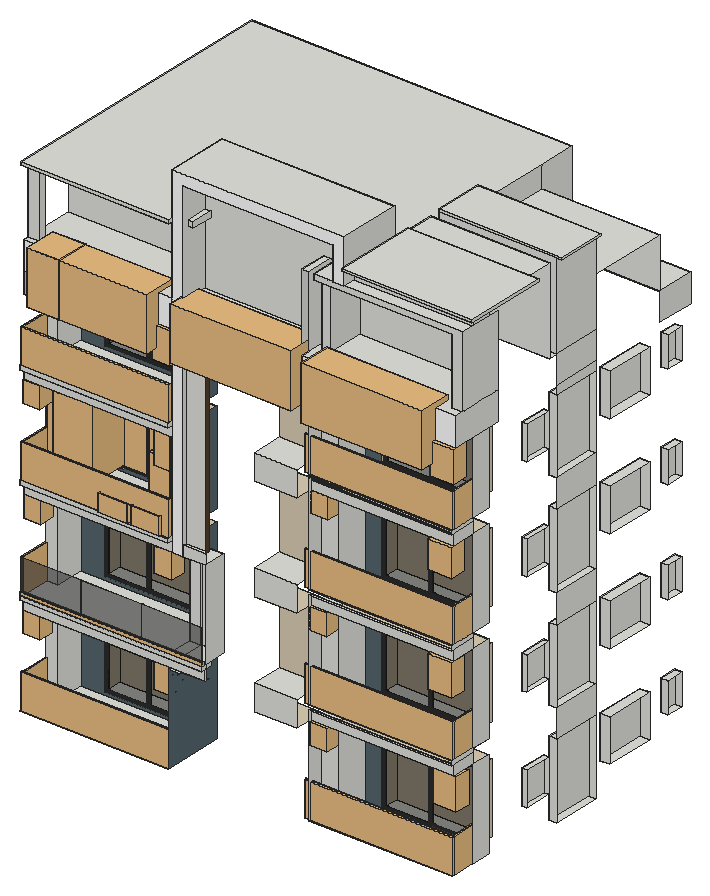
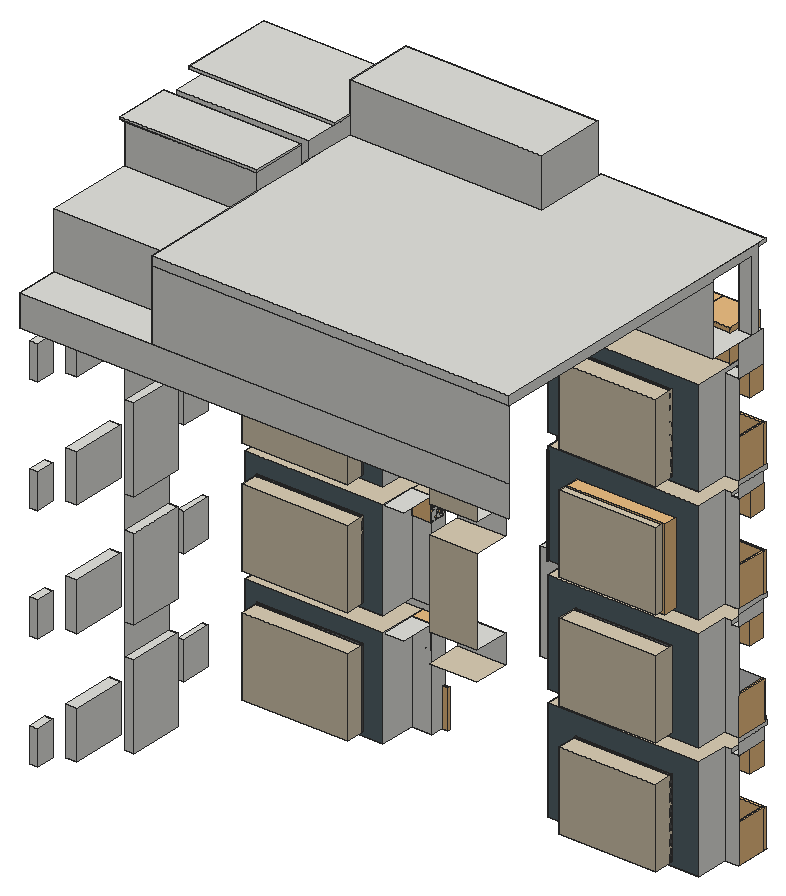
# SketchUp Ruby script. Lengths in inches.
U = 1.inch
M = Sketchup.active_model
def pt(a) = Geom::Point3d.new(a.map { |v| v * U })
def face(e, loops, mat)
  f = e.add_face(loops[0].map { |a| pt(a) })
  loops[1..].each { |l| e.add_face(l.map { |a| pt(a) }).erase! }
  f.material = f.back_material = mat if mat
  f
end
# faces: each face lists its corners as indices into pts; further lists are holes
def faces(e, pts, list, mat = nil) = list.each { |f| face(e, (f[0].is_a?(Array) ? f : [f]).map { |l| l.map { |i| pts[i] } }, mat) }
# xy, xz, yz: faces in a plane at the given z, y or x. An outline is a flat list of corners, or four numbers for a rectangle; further outlines are holes
def ring(l) = l.size == 4 ? [[l[0], l[1]], [l[2], l[1]], [l[2], l[3]], [l[0], l[3]]] : l.each_slice(2).to_a
def flat(e, list, mat, &to3) = list.each { |f| face(e, (f[0].is_a?(Array) ? f : [f]).map { |l| ring(l).map { |u, v| to3.(u, v) } }, mat) }
def xy(e, z, list, mat = nil) = flat(e, list, mat) { |x, y| [x, y, z] }
def xz(e, y, list, mat = nil) = flat(e, list, mat) { |x, z| [x, y, z] }
def yz(e, x, list, mat = nil) = flat(e, list, mat) { |y, z| [x, y, z] }
def lines(e, pts, list) = list.each { |a, b| e.add_line(pt(pts[a]), pt(pts[b])) }
# prism: a flat outline (further loops are holes) pulled along v
def prism(e, loops, v, mat = nil)
  f = face(e, loops, mat); d = Geom::Vector3d.new(v.map { |x| x * U })
  f.pushpull(f.normal.samedirection?(d) ? d.length : -d.length)
end
def box(e, o, s, mat = nil) = prism(e, [[o, [o[0] + s[0], o[1], o[2]], [o[0] + s[0], o[1] + s[1], o[2]], [o[0], o[1] + s[1], o[2]]]], [0, 0, s[2]], mat)
def at(x, y, z, deg = 0) = Geom::Transformation.translation(pt([x, y, z])) * Geom::Transformation.rotation(ORIGIN, Z_AXIS, deg.degrees)
def axes(o, x, y, z) = Geom::Transformation.new([*x, 0, *y, 0, *z, 0, *pt(o).to_a, 1])
def part(name) = M.definitions.add(name)
# library, detail: a bought-in or finely detailed component or shape, given as its bounding box
def library(name, o, s) = part(name).tap { |d| box(d.entities, o, s) }
def detail(e, o, s) = box(e.add_group.entities, o, s)
def put(e, d, t, mat = nil) = e.add_instance(d, t).tap { |i| i.material = mat if mat }
def group(e, t, mat = nil) = e.add_group.tap { |g| g.transformation = t; g.material = mat if mat }.entities
root = M.entities
M.materials.add("Glass_Tinted_Gray").color = [0, 0, 0]
M.materials["Glass_Tinted_Gray"].alpha = 0.125
M.materials.add("Wall Paint Bumpy 01 Blue 100cm").color = [86, 103, 109]
M.materials.add("Wood Planks Pecan 33-81 150cm").color = [83, 63, 40]
M.materials.add("[0135_DarkGray]").color = [81, 81, 81]
M.materials.add("[Color M00]").color = [255, 255, 255]
M.materials.add("[Mirror 02]").color = [96, 96, 96]
M.materials["[Mirror 02]"].alpha = 0.27
M.materials.add("[Terrazzo Light Blue]").color = [196, 214, 227]
M.materials.add("[Translucent_Glass_Blue]").color = [63, 63, 63]
M.materials["[Translucent_Glass_Blue]"].alpha = 0.35
M.materials.add("metal railing").color = [165, 165, 165]
M.materials.add("plastic2").color = [86, 86, 86]
M.materials.add("warmk").color = [218, 205, 180]
c1 = library("My+Glass_Railing\#1",[-0.12,0,0],[177.09,2.52,40.9])
c2 = library("My+Glass_Railing\#5",[-0.02,0,0],[34.55,2.52,40.9])
c3 = library("My+Glass_Railing\#6",[-0.02,0,0],[30.48,2.52,40.9])
c4 = part("PENTEK_RP Fineline 50S_Sliding_DoorCase_E1")
box(c4.entities,[0,0,0],[1.51,3.66,99.27],"[0135_DarkGray]")
c5 = part("PENTEK_RP Fineline 50S_SlidingDooe_Case_E2")
box(c5.entities,[0,0,0],[96.25,3.66,1.51],"[0135_DarkGray]")
c6 = part("pentek_RP Fineline 50S_SlidingDoor_Case")
put(c6.entities,c4,at(97.76,0,0))
put(c6.entities,c5,at(1.51,0,0))
put(c6.entities,c4,at(0,0,0))
put(c6.entities,c5,at(1.51,0,97.76))
c7 = part("PENTEK_RP Fineline 50S_SlidingDoor_GlazingBead_2")
box(c7.entities,[0,0,0],[0.56,0.59,94.39],"[0135_DarkGray]")
c8 = part("PENTEK_RP Fineline 50S_SlidingDoor_GlazingBead")
box(c8.entities,[0,0,0],[45.47,0.59,0.56],"[0135_DarkGray]")
c9 = part("PENTEK_RP Fineline 50S_SlidingDoor_Glass")
box(c9.entities,[0,0,0],[46.58,0.16,94.39],"Glass_Tinted_Gray")
c10 = part("PENTEK_RP Fineline 50S_SlidingDoor_Leaf_E1")
xy(c10.entities,0,[[0,0,0.93,1.97],[0.93,1.57,1.49,1.97]],"[0135_DarkGray]")
xy(c10.entities,96.25,[[0,0,0.93,0,0.93,1.57,1.49,1.57,1.49,1.97,0,1.97]],"[0135_DarkGray]")
xz(c10.entities,0,[[0,0,0.93,96.25]],"[0135_DarkGray]")
xz(c10.entities,1.57,[[0.93,0,1.49,95.32],[0.93,95.32,1.49,96.25]],"[0135_DarkGray]")
xz(c10.entities,1.97,[[0,0,1.49,96.25]],"[0135_DarkGray]")
yz(c10.entities,0,[[0,0,1.97,96.25]],"[0135_DarkGray]")
yz(c10.entities,0.93,[[0,0,1.57,0.93],[0,0.93,1.57,95.32],[0,95.32,1.57,96.25]],"[0135_DarkGray]")
yz(c10.entities,1.49,[[1.57,0,1.97,95.32],[1.57,95.32,1.97,96.25]],"[0135_DarkGray]")
c11 = part("PENTEK_RP Fineline 50S_SlidingDoor_Leaf_E2")
xy(c11.entities,0,[[0,0,0,1.57,0.56,1.57,0.56,1.97,46.02,1.97,46.02,1.57,46.58,1.57,46.58,0]],"[0135_DarkGray]")
xy(c11.entities,0.93,[[0,0,46.58,1.57]],"[0135_DarkGray]")
xy(c11.entities,1.49,[[0.56,1.57,46.02,1.97]],"[0135_DarkGray]")
xz(c11.entities,0,[[0,0,46.58,0.93]],"[0135_DarkGray]")
xz(c11.entities,1.57,[[0,0,0.56,0.93],[46.02,0,46.58,0.93],[0.56,0.93,46.02,1.49]],"[0135_DarkGray]")
xz(c11.entities,1.97,[[0.56,0,46.02,1.49]],"[0135_DarkGray]")
yz(c11.entities,0,[[0,0,1.57,0.93]],"[0135_DarkGray]")
yz(c11.entities,0.56,[[1.57,0,1.97,0.93],[1.57,0.93,1.97,1.49]],"[0135_DarkGray]")
yz(c11.entities,46.02,[[1.57,0,1.97,0.93],[1.57,0.93,1.97,1.49]],"[0135_DarkGray]")
yz(c11.entities,46.58,[[0,0,1.57,0.93]],"[0135_DarkGray]")
c12 = part("PENTEK_RP Fineline S_SlidingDoor_Leaf1")
put(c12.entities,c7,at(0.93,0,0.93))
put(c12.entities,c7,at(46.96,0,0.93))
put(c12.entities,c8,at(1.49,0,0.93))
put(c12.entities,c9,at(1.49,0.59,0.93),"[Terrazzo Light Blue]")
put(c12.entities,c10,at(0,0,0))
put(c12.entities,c10,axes([48.44,0,0],[-1,0,0],[0,1,0],[0,0,1]))
put(c12.entities,c11,axes([0.93,0,96.25],[1,0,0],[0,1,0],[0,0,-1]))
put(c12.entities,c8,at(1.49,0,94.77))
put(c12.entities,c9,at(1.49,1.42,0.93))
put(c12.entities,c11,at(0.93,0,0))
c13 = part("PENTEK_RP Fineline 50S_SlidingDoor_Leaf2")
put(c13.entities,c9,at(1.49,1.42,0.93))
put(c13.entities,c8,at(1.49,0,94.77))
put(c13.entities,c7,at(46.96,0,0.93))
put(c13.entities,c9,at(1.49,0.59,0.93),"[Mirror 02]")
put(c13.entities,c7,at(0.93,0,0.93))
put(c13.entities,c10,at(0,0,0))
put(c13.entities,c10,axes([48.44,0,0],[-1,0,0],[0,1,0],[0,0,1]))
put(c13.entities,c8,at(1.49,0,0.93))
put(c13.entities,c11,axes([0.93,0,96.25],[1,0,0],[0,1,0],[0,0,-1]))
put(c13.entities,c11,at(0.93,0,0))
c14 = part("PENTEK - Slimmest Steel Sliding Door / Window\#1")
put(c14.entities,c6,at(0,-1.88,-0.09))
put(c14.entities,c12,at(1.51,-2.27,1.42),"[Mirror 02]")
put(c14.entities,c13,at(49.32,-0.3,1.42),"[Mirror 02]")
c15 = library("Plante \#58",[-0.43,-1.58,0],[20.84,18.06,17.59])
c16 = library("Railing",[0,0,0],[72,2.52,4.03])
c17 = part("railing plastic")
box(c17.entities,[0,0.75,0],[72,0.26,0.68],"plastic2")
box(c17.entities,[0,0,0],[72,0.26,0.68],"plastic2")
c18 = part("Glass Railing pro\#2")
put(c18.entities,c16,axes([0,0,0],[3.01682,0,0],[0,1,0],[0,0,1]))
put(c18.entities,c17,axes([0,0.75,3.47],[3.01682,0,0],[0,1,0],[0,0,1]))
c19 = part("sheet glass")
box(c19.entities,[0,0,0],[39.37,0.39,39.37],"[Translucent_Glass_Blue]")
c20 = part("glass stretch")
box(c20.entities,[0,0,0],[39.37,0.39,43.31],"[Translucent_Glass_Blue]")
c21 = part("glass frame\#2")
put(c21.entities,c19,axes([0,0,0],[1.8288,0,0],[0,1.016,0],[0,0,1]))
put(c21.entities,c20,axes([216.6,0,0],[0.01552,0,0],[0,1.016,0],[0,0,0.90909]))
put(c21.entities,c19,axes([72.2,0,0],[1.8288,0,0],[0,1.016,0],[0,0,1]))
put(c21.entities,c19,axes([144.4,0,0],[1.8288,0,0],[0,1.016,0],[0,0,1]))
c22 = part("Glass Railing +\#2")
put(c22.entities,c18,at(0,0,0),"metal railing")
put(c22.entities,c21,at(0,1.0625,1.53),"metal railing")
c23 = part("My+Glass_Railing\#2")
put(c23.entities,c22,at(-0.14,0,0))
c24 = library("Scara+cu+plante",[-7.66,-9.41,-0.15],[30.59,22.83,66.38])
c25 = library("Group\#13",[0,0,0],[56.8,25.91,35.15])
c26 = library("Wall Panel 104-13",[-34.04,-0.13,-0.01],[68.11,0.26,99.14])
c27 = library("MODEL",[0,0,0],[31.5,0.12,106.3])
c28 = library("Curtain set",[0,0,0],[14.46,147.43,135.83])
c29 = library("Premium Outdoor Hammock Chair Fern",[-23.82,-23.01,-106.08],[47.64,46.02,106.08])
c30 = library("Grupo1\#1",[206.08,217.32,0],[24.37,24.38,27.75])
c31 = library("climbing plant",[8874.76,-5589.78,-33.625],[50.13,38.07,87.16])
c32 = library("Group\#2",[0,0,0],[143.94,39.08,63.625])
xy(root,628.16,[[0,26.52,176.99,26.52,176.99,99,14.45,99,14.45,64.57,0,64.57],[340.89,32.16,511.32,32.16,511.32,87.39,362.73,87.39,362.73,49.47,340.89,49.47],[515.49,172.42,524.5,231.18]])
xy(root,632.34,[[384.04,87.39,497.86,108.38],[43.39,99,146.83,121.27]])
xy(root,656.28,[[512.56,251.74,524.5,310.65]])
xy(root,664.54,[[518.78,127.53,524.5,159.82]])
xy(root,670.96,[[516.25,338.3,524.5,358.82]])
xy(root,705.11,[[518.78,127.53,524.5,159.82]])
xy(root,707.45,[[512.56,251.74,524.5,310.65]])
xy(root,707.99,[[516.25,338.3,524.5,358.82]])
xy(root,716.125,[[269.54,39.85,320.5,78.02],[384.04,87.39,497.86,108.38],[43.39,99,146.83,121.27]],"warmk")
xy(root,718.13,[[515.49,172.42,524.5,231.18]])
xy(root,734.36,[[176.99,27.71,190.43,30.65],[0,30.65,0,64.57,7.22,64.57,7.22,35.38,176.99,35.38,176.99,30.65],[190.43,30.65,217.21,36.36],[340.89,49.47,362.73,87.39]])
xy(root,734.36,[[340.89,34.48,340.89,49.47,362.73,49.47,362.73,87.39,511.32,87.39,511.32,34.48]],"warmk")
xy(root,737.79,[[7.22,35.38,7.22,64.57,14.45,64.57,14.45,99,176.99,99,176.99,35.38]],"warmk")
xy(root,746.57,[[0,26.52,217.21,30.65],[340.89,32.16,511.32,34.48],[269.54,39.85,320.5,78.02]])
xy(root,751.45,[[0,26.52,176.99,26.52,176.99,99,14.45,99,14.45,64.57,0,64.57],[176.99,26.52,190.43,58.85],[190.43,26.52,217.21,59.71],[340.89,32.16,511.32,32.16,511.32,87.39,362.73,87.39,362.73,49.47,340.89,49.47],[515.49,172.42,524.5,231.18]])
xy(root,755.64,[[384.04,87.39,497.86,108.38],[43.39,99,146.83,121.27]])
xy(root,779.57,[[512.56,251.74,524.5,310.65]])
xy(root,787.83,[[518.78,127.53,524.5,159.82]])
xy(root,794.25,[[516.25,338.3,524.5,358.82]])
xy(root,828.41,[[518.78,127.53,524.5,159.82]])
xy(root,830.75,[[512.56,251.74,524.5,310.65]])
xy(root,831.29,[[516.25,338.3,524.5,358.82]])
xy(root,839.42,[[269.54,39.85,320.5,78.02],[384.04,87.39,497.86,108.38],[43.39,99,146.83,121.27]],"warmk")
xy(root,839.75,[[515.49,172.42,524.5,231.18]])
xy(root,857.66,[[0,31.69,0,64.57,7.22,64.57,7.22,34.98,176.99,34.98,176.99,31.69],[176.99,31.69,176.99,58.85,190.43,58.85,190.43,59.71,217.21,59.71,217.21,32.07,190.43,32.07,190.43,31.69],[340.89,49.47,362.73,87.39]])
xy(root,857.66,[[340.89,34.48,340.89,49.47,362.73,49.47,362.73,87.39,511.32,87.39,511.32,34.48]],"warmk")
xy(root,861.09,[[7.22,34.98,7.22,64.57,14.45,64.57,14.45,99,176.99,99,176.99,34.98]],"warmk")
xy(root,869.87,[[0,26.52,176.99,31.69],[190.43,32.07,217.21,36.36],[340.89,32.16,511.32,34.48],[269.54,39.85,320.5,78.02]])
xy(root,874.75,[[0,26.52,176.99,26.52,176.99,99,14.45,99,14.45,64.57,0,64.57],[340.89,32.16,511.32,32.16,511.32,87.39,362.73,87.39,362.73,49.47,340.89,49.47],[515.49,172.42,524.5,231.18]])
xy(root,878.93,[[384.04,87.39,497.86,108.38],[43.39,99,146.83,121.27]])
xy(root,902.87,[[512.56,251.74,524.5,310.65]])
xy(root,911.13,[[518.78,127.53,524.5,159.82]])
xy(root,917.55,[[516.25,338.3,524.5,358.82]])
xy(root,951.7,[[518.78,127.53,524.5,159.82]])
xy(root,954.05,[[512.56,251.74,524.5,310.65]])
xy(root,954.59,[[516.25,338.3,524.5,358.82]])
xy(root,962.72,[[269.54,39.85,320.5,78.02],[384.04,87.39,497.86,108.38],[43.39,99,146.83,121.27]],"warmk")
xy(root,964.73,[[515.49,172.42,524.5,231.18]])
xy(root,980.96,[[0,31.69,0,64.57,7.22,64.57,7.22,34.98,176.99,34.98,176.99,31.69],[340.89,49.47,362.73,87.39]])
xy(root,980.96,[[340.89,34.48,340.89,49.47,362.73,49.47,362.73,87.39,511.32,87.39,511.32,34.48]],"warmk")
xy(root,984.38,[[7.22,34.98,7.22,64.57,14.45,64.57,14.45,99,176.99,99,176.99,34.98]],"warmk")
xy(root,993.17,[[0,26.52,176.99,31.69],[340.89,32.16,511.32,34.48],[269.54,39.85,320.5,78.02]])
xy(root,998.05,[[0,26.52,176.99,26.52,176.99,99,14.45,99,14.45,64.57,0,64.57],[340.89,32.16,511.32,32.16,511.32,87.39,362.73,87.39,362.73,49.47,340.89,49.47],[515.49,172.42,524.5,231.18]])
xy(root,1002.23,[[384.04,87.39,497.86,108.38],[43.39,99,146.83,121.27]])
xy(root,1026.17,[[512.56,251.74,524.5,310.65]])
xy(root,1034.43,[[518.78,127.53,524.5,159.82]])
xy(root,1040.85,[[516.25,338.3,524.5,358.82]])
xy(root,1075,[[518.78,127.53,524.5,159.82]])
xy(root,1077.35,[[512.56,251.74,524.5,310.65]])
xy(root,1077.89,[[516.25,338.3,524.5,358.82]])
xy(root,1082.38,[[269.54,34.48,320.5,78.02]],"warmk")
xy(root,1086.02,[[384.04,87.39,497.86,108.38],[43.39,99,146.83,121.27]],"warmk")
xy(root,1086.35,[[515.49,172.42,524.5,231.18]])
xy(root,1096.46,[[0,31.69,0,64.57,14.45,64.57,14.45,40.42,176.99,40.42,176.99,31.69],[258.12,34.48,320.5,36.36],[320.5,34.48,332.22,36.36]])
xy(root,1096.46,[[217.21,32.07,258.12,36.36]],"Wood Planks Pecan 33-81 150cm")
xy(root,1096.46,[[340.89,20.92,340.89,49.47,362.73,49.47,362.73,87.39,511.32,87.39,511.32,63.53,524.5,63.53,524.5,20.92]],"warmk")
xy(root,1100.36,[[14.45,40.42,176.99,99]],"warmk")
xy(root,1130.13,[[340.89,20.92,524.5,20.92,524.5,31.69,511.32,31.69,511.32,87.39,357.79,87.39,357.79,43.39,346.54,43.39,346.54,87.39,340.89,87.39],[0,31.69,176.99,31.69,176.99,99,0,99,0,46.33,14.45,46.33,14.45,38.86,0,38.86],[190.43,36.36,332.22,65.06],[346.54,43.39,357.79,87.39],[383,161.36,524.5,172.42],
  [383,326.45,524.5,372.25]])
xy(root,1189.91,[[383,231.18,524.5,326.45]])
xy(root,1206,[[14.45,38.86,176.99,48.17],[0,46.33,14.45,99]])
xy(root,1208.32,[[190.43,38.86,197.04,65.06],[14.45,48.17,176.99,99]])
xy(root,1208.4375,[[346.54,31.69,346.54,43.39,357.79,43.39,357.79,87.39,511.32,87.39,511.32,31.69]])
xy(root,1211.28,[[0,27.71,176.99,38.86]])
xy(root,1215.07,[[0,27.71,176.99,27.71,176.99,106.96,383,106.96,383,372.25,0,372.25],[346.54,31.69,369.83,65.06],[383,31.69,524.5,46.41],[332.22,32.16,340.89,65.06],[190.43,38.86,197.04,65.06],
  [340.89,65.06,346.54,87.39]])
xy(root,1232.51,[[383,27.71,383,46.41,524.5,46.41,524.5,127.53,538.96,127.53,538.96,27.71],[383,46.41,524.5,127.53],[383,127.53,524.5,161.36],[383,172.42,524.5,231.18],[524.5,172.42,530.47,231.18]])
xy(root,1235.17,[[383,27.71,538.96,127.53],[383,172.42,530.47,231.18]])
xy(root,1254.26,[[190.43,31.69,369.83,65.06]])
xy(root,1267.21,[[176.99,31.69,383,106.96]])
xz(root,20.92,[[340.89,1096.46,524.5,1130.13]],"[Color M00]")
xz(root,26.52,[[0,746.57,217.21,751.45],[0,869.87,176.99,874.75],[0,993.17,176.99,998.05]])
xz(root,27.71,[[0,1211.28,176.99,1215.07],[383,1232.51,538.96,1235.17]])
xz(root,30.65,[[0,734.36,217.21,746.57]])
xz(root,31.69,[[0,857.66,176.99,869.87],[0,980.96,176.99,993.17],[511.32,1130.13,524.5,1130.13,524.5,1215.07,346.54,1215.07,346.54,1208.4375,511.32,1208.4375]])
xz(root,31.69,[[176.99,857.66,190.43,857.66,190.43,1254.26,369.83,1254.26,369.83,1215.07,383,1215.07,383,1267.21,176.99,1267.21],[0,1096.46,176.99,1130.13]],"[Color M00]")
xz(root,32.07,[[190.43,857.66,217.21,869.87]])
xz(root,34.48,[[340.89,734.36,511.32,746.57],[340.89,857.66,511.32,869.87],[340.89,980.96,511.32,993.17]])
xz(root,34.98,[[7.22,857.66,176.99,861.09],[7.22,980.96,176.99,984.38]])
xz(root,35.38,[[7.22,734.36,176.99,737.79]])
xz(root,36.36,[[190.43,869.87,217.21,869.87,217.21,1096.46,332.22,1096.46,332.22,1130.13,190.43,1130.13]])
xz(root,38.86,[[0,1130.13,14.45,1130.13,14.45,1206,176.99,1206,176.99,1211.28,0,1211.28],[190.43,1208.32,197.04,1215.07]])
xz(root,39.85,[[269.54,716.125,320.5,746.57],[269.54,839.42,320.5,869.87],[269.54,962.72,320.5,993.17]])
xz(root,40.42,[[14.45,1096.46,176.99,1100.36]])
xz(root,43.39,[[346.54,1130.13,357.79,1208.4375]])
xz(root,46.33,[[0,1130.13,14.45,1206]])
xz(root,46.41,[[383,1215.07,524.5,1232.51]])
xz(root,48.17,[[14.45,1206,176.99,1208.32]])
xz(root,49.47,[[340.89,628.16,362.73,734.36],[340.89,751.45,362.73,857.66],[340.89,874.75,362.73,980.96],[340.89,998.05,362.73,1096.46]])
xz(root,58.85,[[176.99,751.45,190.43,857.66]])
xz(root,59.71,[[190.43,751.45,217.21,857.66]])
xz(root,64.57,[[0,628.16,14.45,628.16,14.45,737.79,7.22,737.79,7.22,734.36,0,734.36],[0,751.45,14.45,751.45,14.45,861.09,7.22,861.09,7.22,857.66,0,857.66],[0,874.75,14.45,874.75,14.45,984.38,7.22,984.38,7.22,980.96,0,980.96],[0,998.05,14.45,1096.46]])
xz(root,65.06,[[190.43,1130.13,332.22,1130.13,332.22,1215.07,369.83,1215.07,369.83,1254.26,190.43,1254.26,190.43,1215.07,197.04,1215.07,197.04,1208.32,190.43,1208.32]])
xz(root,78.02,[[269.54,746.57,320.5,839.42],[269.54,869.87,320.5,962.72],[269.54,993.17,320.5,1082.38]],"warmk")
xz(root,87.39,[[340.89,1130.13,346.54,1215.07],[357.79,1130.13,511.32,1208.4375]])
xz(root,87.39,[[[362.73,628.16,511.32,734.36],[384.04,632.34,497.86,716.125]],[[362.73,751.45,511.32,857.66],[384.04,755.64,497.86,839.42]],[[362.73,874.75,511.32,980.96],[384.04,878.93,497.86,962.72]],[[362.73,998.05,511.32,1096.46],[384.04,1002.23,497.86,1086.02]]],"Wall Paint Bumpy 01 Blue 100cm")
xz(root,99,[[0,1130.13,176.99,1130.13,176.99,1208.32,14.45,1208.32,14.45,1206,0,1206]])
xz(root,99,[[[14.45,628.16,176.99,737.79],[43.39,632.34,146.83,716.125]],[[14.45,751.45,176.99,861.09],[43.39,755.64,146.83,839.42]],[[14.45,874.75,176.99,984.38],[43.39,878.93,146.83,962.72]],[[14.45,998.05,176.99,1100.36],[43.39,1002.23,146.83,1086.02]]],"Wall Paint Bumpy 01 Blue 100cm")
xz(root,106.96,[[176.99,1215.07,383,1267.21]])
xz(root,108.38,[[384.04,632.34,497.86,716.125],[384.04,755.64,497.86,839.42],[384.04,878.93,497.86,962.72],[384.04,1002.23,497.86,1086.02]],"warmk")
xz(root,121.27,[[43.39,632.34,146.83,716.125],[43.39,755.64,146.83,839.42],[43.39,878.93,146.83,962.72],[43.39,1002.23,146.83,1086.02]],"warmk")
xz(root,127.53,[[518.78,664.54,524.5,705.11],[518.78,787.83,524.5,828.41],[518.78,911.13,524.5,951.7],[518.78,1034.43,524.5,1075],[383,1232.51,538.96,1235.17]])
xz(root,159.82,[[518.78,664.54,524.5,705.11],[518.78,787.83,524.5,828.41],[518.78,911.13,524.5,951.7],[518.78,1034.43,524.5,1075]])
xz(root,161.36,[[383,1130.13,524.5,1232.51]])
xz(root,172.42,[[515.49,628.16,524.5,718.13],[515.49,751.45,524.5,839.75],[515.49,874.75,524.5,964.73],[515.49,998.05,524.5,1086.35],[383,1130.13,524.5,1232.51],
  [383,1232.51,530.47,1235.17]])
xz(root,231.18,[[515.49,628.16,524.5,718.13],[515.49,751.45,524.5,839.75],[515.49,874.75,524.5,964.73],[515.49,998.05,524.5,1086.35],[383,1189.91,524.5,1232.51],
  [383,1232.51,530.47,1235.17]])
xz(root,251.74,[[512.56,656.28,524.5,707.45],[512.56,779.57,524.5,830.75],[512.56,902.87,524.5,954.05],[512.56,1026.17,524.5,1077.35]])
xz(root,310.65,[[512.56,656.28,524.5,707.45],[512.56,779.57,524.5,830.75],[512.56,902.87,524.5,954.05],[512.56,1026.17,524.5,1077.35]])
xz(root,326.45,[[383,1130.13,524.5,1189.91]])
xz(root,338.3,[[516.25,670.96,524.5,707.99],[516.25,794.25,524.5,831.29],[516.25,917.55,524.5,954.59],[516.25,1040.85,524.5,1077.89]])
xz(root,358.82,[[516.25,670.96,524.5,707.99],[516.25,794.25,524.5,831.29],[516.25,917.55,524.5,954.59],[516.25,1040.85,524.5,1077.89]])
xz(root,372.25,[[0,1096.46,524.5,1130.13],[0,1130.13,383,1204.84],[0,1204.84,383,1215.07]])
yz(root,0,[[30.65,734.36,64.57,746.57],[26.52,746.57,64.57,751.45],[31.69,857.66,64.57,869.87],[26.52,869.87,64.57,874.75],[31.69,980.96,64.57,993.17],
  [26.52,993.17,64.57,998.05],[31.69,1096.46,64.57,1130.13],[38.86,1130.13,38.86,1215.07,372.25,1215.07,372.25,1204.84,99,1204.84,99,1206,46.33,1206,46.33,1130.13],[27.71,1211.28,38.86,1215.07]])
yz(root,7.22,[[35.38,734.36,64.57,737.79],[34.98,857.66,64.57,861.09],[34.98,980.96,64.57,984.38]])
yz(root,14.45,[[64.57,628.16,99,737.79],[64.57,751.45,99,861.09],[64.57,874.75,99,984.38],[64.57,998.05,99,998.05,99,1100.36,40.42,1100.36,40.42,1096.46,64.57,1096.46],[38.86,1130.13,46.33,1206],
  [48.17,1206,99,1208.32]])
yz(root,43.39,[[99,632.34,121.27,716.125],[99,755.64,121.27,839.42],[99,878.93,121.27,962.72],[99,1002.23,121.27,1086.02]],"warmk")
yz(root,146.83,[[99,632.34,121.27,716.125],[99,755.64,121.27,839.42],[99,878.93,121.27,962.72],[99,1002.23,121.27,1086.02]],"warmk")
yz(root,176.99,[[34.98,857.66,58.85,861.09],[26.52,869.87,31.69,874.75],[26.52,993.17,31.69,998.05],[31.69,1130.13,31.69,1208.32,38.86,1208.32,38.86,1206,48.17,1206,48.17,1208.32,99,1208.32,99,1130.13],[31.69,1208.32,38.86,1211.28],
  [27.71,1211.28,31.69,1215.07],[31.69,1215.07,106.96,1267.21]])
yz(root,176.99,[[27.71,628.16,27.71,734.36,35.38,734.36,35.38,737.79,99,737.79,99,628.16],[58.85,751.45,99,861.09],[31.69,874.75,31.69,980.96,34.98,980.96,34.98,984.38,99,984.38,99,874.75],[31.69,998.05,31.69,1096.46,40.42,1096.46,40.42,1100.36,99,1100.36,99,998.05]],"Wall Paint Bumpy 01 Blue 100cm")
yz(root,190.43,[[58.85,751.45,59.71,857.66],[31.69,857.66,32.07,869.87],[31.69,869.87,36.36,1130.13],[31.69,1130.13,65.06,1130.13,65.06,1208.32,38.86,1208.32,38.86,1215.07,65.06,1215.07,65.06,1254.26,31.69,1254.26]])
yz(root,197.04,[[38.86,1208.32,65.06,1215.07]])
yz(root,217.21,[[30.65,734.36,32.07,746.57],[26.52,746.57,32.07,751.45],[32.07,746.57,39.41,751.45],[32.07,751.45,59.71,857.66]])
yz(root,217.21,[[32.07,869.87,36.36,1096.46]],"Wood Planks Pecan 33-81 150cm")
yz(root,332.22,[[32.16,1096.46,36.36,1130.13],[32.16,1130.13,65.06,1215.07]])
yz(root,340.89,[[32.16,628.16,49.47,628.16,49.47,734.36,34.48,734.36,34.48,746.57,32.16,746.57],[32.16,751.45,49.47,751.45,49.47,857.66,34.48,857.66,34.48,869.87,32.16,869.87],[32.16,874.75,49.47,874.75,49.47,980.96,34.48,980.96,34.48,993.17,32.16,993.17],[32.16,998.05,49.47,1096.46],[20.92,1096.46,32.16,1130.13],
  [32.16,1130.13,87.39,1215.07]])
yz(root,346.54,[[43.39,1130.13,87.39,1208.4375],[31.69,1208.4375,43.39,1215.07],[43.39,1208.4375,87.39,1215.07]])
yz(root,357.79,[[43.39,1130.13,87.39,1208.4375]])
yz(root,362.73,[[49.47,628.16,87.39,734.36],[49.47,751.45,87.39,857.66],[49.47,874.75,87.39,980.96],[49.47,998.05,87.39,1096.46]])
yz(root,369.83,[[31.69,1215.07,65.06,1254.26]])
yz(root,383,[[161.36,1130.13,172.42,1215.07],[326.45,1130.13,372.25,1215.07],[231.18,1189.91,326.45,1215.07],[31.69,1215.07,46.41,1232.51],[106.96,1215.07,161.36,1232.51],
  [172.42,1215.07,231.18,1232.51],[27.71,1232.51,31.69,1235.17],[31.69,1232.51,106.96,1235.17],[106.96,1232.51,127.53,1235.17],[172.42,1232.51,231.18,1235.17],
  [31.69,1235.17,106.96,1267.21]])
yz(root,384.04,[[87.39,632.34,108.38,716.125],[87.39,755.64,108.38,839.42],[87.39,878.93,108.38,962.72],[87.39,1002.23,108.38,1086.02]],"warmk")
yz(root,497.86,[[87.39,632.34,108.38,716.125],[87.39,755.64,108.38,839.42],[87.39,878.93,108.38,962.72],[87.39,1002.23,108.38,1086.02]],"warmk")
yz(root,511.32,[[63.53,628.16,87.39,734.36],[34.48,734.36,63.53,746.57],[32.16,746.57,63.53,751.45],[63.53,751.45,87.39,857.66],[34.48,857.66,63.53,869.87],
  [32.16,869.87,63.53,874.75],[63.53,874.75,87.39,980.96],[34.48,980.96,63.53,993.17],[32.16,993.17,63.53,998.05],[63.53,998.05,87.39,1096.46],
  [31.69,1130.13,87.39,1208.4375]])
yz(root,512.56,[[251.74,656.28,310.65,707.45],[251.74,779.57,310.65,830.75],[251.74,902.87,310.65,954.05],[251.74,1026.17,310.65,1077.35]])
yz(root,515.49,[[172.42,628.16,231.18,718.13],[172.42,751.45,231.18,839.75],[172.42,874.75,231.18,964.73],[172.42,998.05,231.18,1086.35]])
yz(root,516.25,[[338.3,670.96,358.82,707.99],[338.3,794.25,358.82,831.29],[338.3,917.55,358.82,954.59],[338.3,1040.85,358.82,1077.89]])
yz(root,518.78,[[127.53,664.54,159.82,705.11],[127.53,787.83,159.82,828.41],[127.53,911.13,159.82,951.7],[127.53,1034.43,159.82,1075]])
yz(root,524.5,[[172.42,718.13,231.18,751.45],[172.42,839.75,231.18,874.75],[172.42,964.73,231.18,998.05],[172.42,1086.35,231.18,1096.46],[20.92,1096.46,84.62,1130.13],
  [172.42,1096.46,231.18,1130.13],[326.45,1096.46,372.25,1130.13],[31.69,1130.13,84.62,1215.07],[172.42,1130.13,231.18,1232.51]])
yz(root,530.47,[[172.42,1232.51,231.18,1235.17]])
yz(root,538.96,[[27.71,1232.51,127.53,1235.17]])
p = [[176.99,39.41,734.36],[190.43,39.41,734.36],[190.43,36.36,734.36],[320.5,36.47,1096.46],[320.5,36.47,1082.38],[340.89,65.06,1204.84],
  [332.22,65.06,1204.84],[320.5,36.36,1096.46]]
lines(root,p,[[0,1],[1,2],[3,4],[5,6],[7,3]])
put(root,c1,at(0.02,27.5,628.16))
put(root,c2,at(2.71,28.99,628.16,90))
put(root,c1,at(334.34,33.63,628.16))
put(root,c3,at(511.32,36.23,628.16,90))
put(root,c14,axes([43.39,100.55,632.42],[1.04197,0,0],[0,0.6832,0],[0,0,0.84587]))
put(root,c14,axes([384.04,88.68,632.7],[1.14656,0,0],[0,0.6832,0],[0,0,0.84587]))
put(root,c15,axes([487.2,36.05,696.9],[1.35,0,0],[0,1,0],[0,0,2.13]))
put(root,c15,axes([156.58,32.23,704.77],[1,0,0],[0,1,0],[0,0,1.6827]))
put(root,c15,axes([342.32,32.99,709.39],[1,0,0],[0,1,0],[0,0,1.42]))
put(root,c15,axes([0.43,32.23,709.39],[1,0,0],[0,1,0],[0,0,1.42]))
put(root,c1,at(334.34,33.63,751.45))
put(root,c23,at(0.14,27.09,751.45))
put(root,c2,at(2.51,29.59,751.45,90))
put(root,c3,at(511.32,36.23,751.45,90))
put(root,c14,axes([43.39,100.55,755.71],[1.04197,0,0],[0,0.6832,0],[0,0,0.84587]))
put(root,c14,axes([384.04,88.68,755.99],[1.14656,0,0],[0,0.6832,0],[0,0,0.84587]))
put(root,c15,axes([484.82,32.29,820.05],[1.35,0,0],[0,1,0],[0,0,2.13]))
put(root,c15,axes([156.58,33.27,828.0625],[1,0,0],[0,1,0],[0,0,1.6827]))
put(root,c15,axes([341.32,34.05,832.05],[1,0,0],[0,1,0],[0,0,1.42]))
put(root,c15,axes([0.43,33.27,832.68],[1,0,0],[0,1,0],[0,0,1.42]))
put(root,c24,axes([143.97,69.11,874.75],[1.38,0,0],[0,1.77,0],[0,0,1]))
put(root,c1,at(334.34,33.63,874.74))
put(root,c25,axes([128.16,25.22,874.75],[0.69,0,0],[0,0.8,0],[0,0,0.57]))
put(root,c25,axes([94.41,25.22,874.75],[0.69,0,0],[0,0.8,0],[0,0,0.57]))
put(root,c1,at(0.02,27.5,874.75))
put(root,c2,at(2.71,28.99,874.75,90))
put(root,c26,axes([176.21,65.73,874.76],[0,1,0],[-6,0,0],[0,0,1.07121]))
put(root,c3,at(511.32,36.23,874.75,90))
put(root,c27,at(2.5,63.52,874.76))
put(root,c28,axes([145.25,99,877.23],[0,1,0],[-0.71772,0,0],[0,0,0.64]))
put(root,c14,axes([43.39,100.55,879.01],[1.04197,0,0],[0,0.6832,0],[0,0,0.84587]))
put(root,c14,axes([384.04,88.68,879.29],[1.14656,0,0],[0,0.6832,0],[0,0,0.84587]))
put(root,c29,axes([58.9,54.7,980.96],[1,0,0],[0,1,0],[0,0,0.784]))
put(root,c15,axes([156.58,33.27,943.5],[1,0,0],[0,1,0],[0,0,2.13]))
put(root,c15,axes([484.82,32.29,947.84],[1.35,0,0],[0,1,0],[0,0,1.8744]))
put(root,c15,axes([341.32,36.05,955.98],[1,0,0],[0,1,0],[0,0,1.42]))
put(root,c15,axes([0.41,31.93,955.98],[1,0,0],[0,1,0],[0,0,1.42]))
put(root,c30,axes([-109.03,-155.67,965.79],[1,0,0],[0,1,0],[0,0,0.67]))
put(root,c1,at(334.34,33.63,998.03))
put(root,c1,at(0.02,27.5,998.05))
put(root,c2,at(2.71,28.99,998.05,90))
put(root,c3,at(511.32,36.23,998.05,90))
put(root,c14,axes([43.39,100.55,1002.31],[1.04197,0,0],[0,0.6832,0],[0,0,0.84587]))
put(root,c14,axes([385.77,88.68,1002.31],[1.14656,0,0],[0,0.6832,0],[0,0,0.84587]),"[Mirror 02]")
put(root,c15,axes([498,18.74,1058.85],[1.35,0,0],[0,1,0],[0,0,2.13]))
put(root,c15,axes([156.96,29.51,1058.85],[1,0,0],[0,1,0],[0,0,2.13]))
put(root,c31,axes([-6905.3125,5753.52,1095.85],[0.78,0,0],[0,1.0266,0],[0,0,0.73]))
put(root,c32,at(17,15.05,1071.31))
put(root,c32,at(188.5,15.05,1071.31))
put(root,c15,axes([341.32,22.5,1071.49],[1,0,0],[0,1,0],[0,0,1.42]))
put(root,c15,axes([0.43,33.27,1071.49],[1,0,0],[0,1,0],[0,0,1.42]))
put(root,c32,at(355.7,1.56,1072.27))
